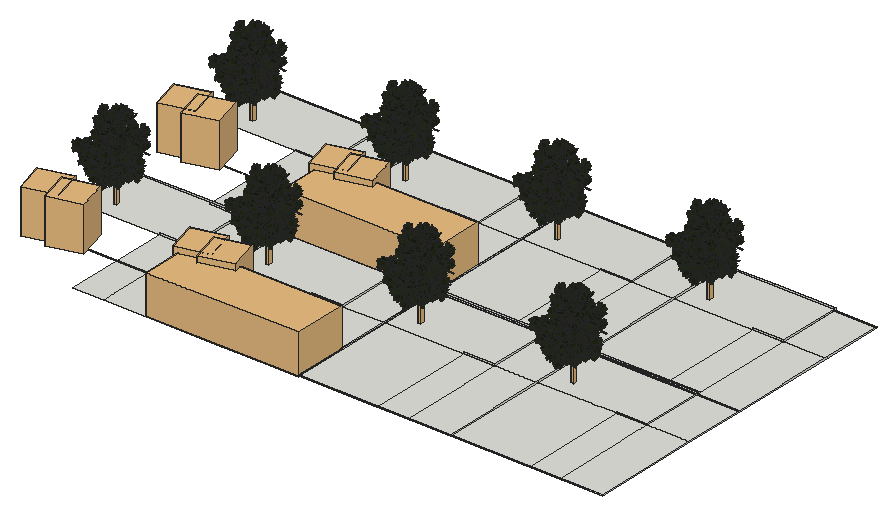
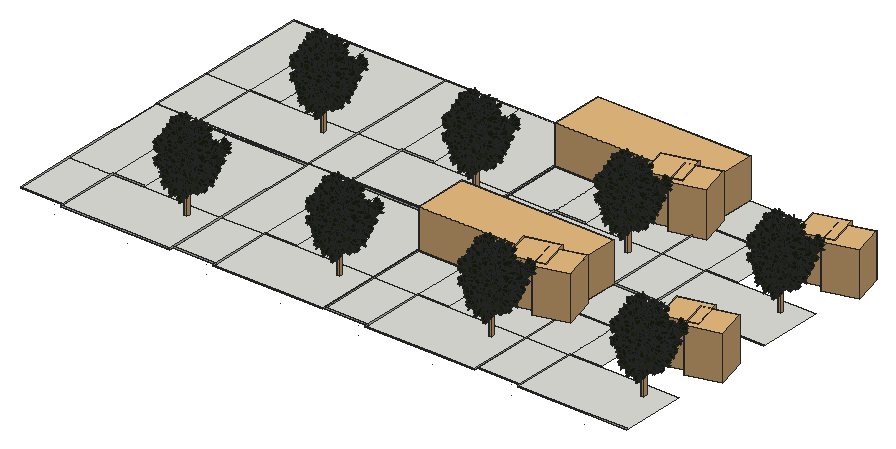
# SketchUp Ruby script. Lengths in inches.
U = 1.inch
M = Sketchup.active_model
def pt(a) = Geom::Point3d.new(a.map { |v| v * U })
def face(e, loops, mat)
  f = e.add_face(loops[0].map { |a| pt(a) })
  loops[1..].each { |l| e.add_face(l.map { |a| pt(a) }).erase! }
  f.material = f.back_material = mat if mat
  f
end
# faces: each face lists its corners as indices into pts; further lists are holes
def faces(e, pts, list, mat = nil) = list.each { |f| face(e, (f[0].is_a?(Array) ? f : [f]).map { |l| l.map { |i| pts[i] } }, mat) }
# xy, xz, yz: faces in a plane at the given z, y or x. An outline is a flat list of corners, or four numbers for a rectangle; further outlines are holes
def ring(l) = l.size == 4 ? [[l[0], l[1]], [l[2], l[1]], [l[2], l[3]], [l[0], l[3]]] : l.each_slice(2).to_a
def flat(e, list, mat, &to3) = list.each { |f| face(e, (f[0].is_a?(Array) ? f : [f]).map { |l| ring(l).map { |u, v| to3.(u, v) } }, mat) }
def xy(e, z, list, mat = nil) = flat(e, list, mat) { |x, y| [x, y, z] }
def xz(e, y, list, mat = nil) = flat(e, list, mat) { |x, z| [x, y, z] }
def yz(e, x, list, mat = nil) = flat(e, list, mat) { |y, z| [x, y, z] }
def lines(e, pts, list) = list.each { |a, b| e.add_line(pt(pts[a]), pt(pts[b])) }
# prism: a flat outline (further loops are holes) pulled along v
def prism(e, loops, v, mat = nil)
  f = face(e, loops, mat); d = Geom::Vector3d.new(v.map { |x| x * U })
  f.pushpull(f.normal.samedirection?(d) ? d.length : -d.length)
end
def box(e, o, s, mat = nil) = prism(e, [[o, [o[0] + s[0], o[1], o[2]], [o[0] + s[0], o[1] + s[1], o[2]], [o[0], o[1] + s[1], o[2]]]], [0, 0, s[2]], mat)
def at(x, y, z, deg = 0) = Geom::Transformation.translation(pt([x, y, z])) * Geom::Transformation.rotation(ORIGIN, Z_AXIS, deg.degrees)
def axes(o, x, y, z) = Geom::Transformation.new([*x, 0, *y, 0, *z, 0, *pt(o).to_a, 1])
def part(name) = M.definitions.add(name)
# library, detail: a bought-in or finely detailed component or shape, given as its bounding box
def library(name, o, s) = part(name).tap { |d| box(d.entities, o, s) }
def detail(e, o, s) = box(e.add_group.entities, o, s)
def put(e, d, t, mat = nil) = e.add_instance(d, t).tap { |i| i.material = mat if mat }
def group(e, t, mat = nil) = e.add_group.tap { |g| g.transformation = t; g.material = mat if mat }.entities
root = M.entities
M.materials.add("Green ash – green texture").color = [33, 41, 22]
M.materials.add("[Color_005]").color = [114, 114, 114]
M.materials.add("[Color_D09]").color = [86, 59, 49]
c1 = part("Component\#22")
xz(c1.entities,0,[[2.54,0,9.87,0.64,10.99,2.07,11.4,3.42,15.13,2.28,14.48,4.31,16.14,5.21,16.14,6.08,19.81,7.28,19.6,9.67,17.45,11.49,17.45,12.16,18.82,14.37,17.48,14.37,14.41,13.66,14.41,15.23,12.5625,17.49,9.84,15.21,8.9,13.85,7.74,13.625,7.35,12.68,6.87,13.02,6.35,12.27,5.92,10.47,4.2,7.42,2.84,6.89,0,2.38,0.07,1.59,2.8125,4.94,3.37,3.59,2.54,3.37,2.12,2.22]],"Green ash – green texture")
c2 = part("Component\#21")
xz(c2.entities,0,[[1.1,0,1.61,0,2.73,1.11,4.34,2.72,5.21,6.36,5.85,7.16,6.35,6.9375,6.85,8.05,8.03,8.05,8.625,9.25,10.11,11.7,9.56,13.83,9.56,15.84,7.83,15.84,6.03,14.37,5.31,16.54,4.4375,17.39,1.45,14.31,0,9.15,1.4,5.18,3.01,6.08,1.98,1.39]],"Green ash – green texture")
c3 = part("Component\#23")
put(c3.entities,c1,axes([0,7.77,0],[1,0,0],[0,0.89571,0.44464],[0,-0.44464,0.89571]))
put(c3.entities,c2,axes([2.15,6.37,5.26],[0.57629,-0.80824,0.12095],[0.79263,0.51673,-0.3236],[0.19905,0.28236,0.93843]))
c4 = part("Component\#24")
put(c4.entities,c3,axes([-4.97,-3.22,4.05],[0.69883,-0.69034,0.18725],[0.53248,0.3273,-0.7806],[0.47759,0.64522,0.59632]))
c5 = part("Component\#25")
put(c5.entities,c4,axes([0,5.2,2.2],[1,0,0],[0,0.90259,0.43051],[0,-0.43051,0.90259]))
c6 = part("leaf group 2")
put(c6.entities,c5,axes([-11.99,4.41,-4.35],[2.22014,-0.82385,1.14017],[1.36501,1.77637,-1.37441],[-0.33979,1.75315,1.92841]))
c7 = part("Component\#28")
put(c7.entities,c6,axes([-5.27,11.65,1.68],[-0.48323,0.10636,-0.43072],[-0.11515,-0.64511,-0.03012],[-0.42845,0.05342,0.49388]))
c8 = part("Component\#27")
xz(c8.entities,0,[[0.64,0,0,0.1875,4.21,2.81,8.59,4.11,12.8,4.11,19.57,2.81,12.8,3.73,8.59,3.73,4.21,2.3125]],"[Color_D09]")
c9 = part("Leafy twig \#1")
put(c9.entities,c7,axes([23.53,12.57,24.85],[0.06536,-0.90475,-0.42089],[0.61791,-0.2945,0.72901],[-0.78353,-0.30772,0.53981]))
put(c9.entities,c7,axes([22.7,12.25,24.83],[-0.47146,-0.89493,0.11311],[0.80135,-0.48549,-0.35888],[0.36776,-0.0521,0.90651]))
put(c9.entities,c7,axes([24.25,0.65,20.83],[0.8253,-0.50372,0.24924],[0.23848,0.71461,0.65749],[-0.51157,-0.48438,0.71194]))
put(c9.entities,c7,axes([23.54,-2.45,18.63],[0.04689,-0.92492,0.3511],[0.72122,-0.28285,-0.64421],[0.71641,0.2674,0.65188]))
put(c9.entities,c7,axes([22.39,16.15,27.04],[-0.5311,-0.82173,0.2419],[0.41574,0.01583,0.89559],[-0.77461,0.50499,0.40813]))
put(c9.entities,c8,axes([22.76,-5.09,13.48],[0,1.66539,0.44624],[-1.72414,0,0],[0,-0.44624,1.66539]))
c10 = part("Component\#26")
p = [[0,0,0.13],[0.41,0.77,0],[4.07,2.79,10.125],[3.73,2.15,10.23],[7.66,4.77,23.875],[7.4,4.27,23.96],
  [8.6875,5.26,35.99],[8.5,4.91,36.05],[8.32,4.9375,46.95],[8.21,4.74,46.98]]
faces(c10.entities,p,[[0,1,2,3],[3,2,4,5],[4,6,7,5],[6,8,9,7]],"[Color_005]")
c11 = part("Component\#30")
put(c11.entities,c10,axes([3.13,0.17,-0.45],[3.38032,6.88592,0.52481],[-5.85488,3.97559,0.303],[0,-1.35912,3.54524]))
put(c11.entities,c7,axes([0.37,31.375,148.94],[0.47772,0.64064,-1.51139],[2.85768,-0.62659,0.20284],[-0.43926,-3.3797,-0.3241]))
c12 = part("Leafy branch")
put(c12.entities,c9,axes([28.11,72.66,46.26],[0.77413,-0.41274,-0.47998],[0.6311,0.56229,0.53435],[0.04934,-0.71657,0.69577]))
put(c12.entities,c9,axes([31.25,3.94,9.17],[0.73236,0.67893,0.05208],[-0.46223,0.55185,-0.69413],[-0.5,0.48428,0.71797]))
put(c12.entities,c9,axes([20.16,84.84,57.95],[0.96628,0.19619,0.16678],[-0.2575,0.73909,0.62245],[-0.00115,-0.6444,0.76469]))
put(c12.entities,c9,axes([30.13,29.18,11.93],[0.86603,0.2796,0.41452],[0,0.82904,-0.55919],[-0.5,0.48428,0.71797]))
put(c12.entities,c9,axes([47.67,28.63,-3.7],[0.1205,-0.71255,0.69119],[0.96646,0.24327,0.08231],[-0.2268,0.65809,0.71797]))
put(c12.entities,c9,axes([48.76,50.64,76.31],[-0.6716,0.46861,-0.57389],[0.01402,0.78248,0.62252],[0.74078,0.41004,-0.53209]))
put(c12.entities,c11,axes([42.34,0,10.34],[0.39368,0,0],[0,0.22544,-0.24092],[0,0.54032,0.50562]))
put(c12.entities,c9,axes([64.51,80.82,101.08],[-0.99604,0.06562,-0.06004],[-0.0106,0.58266,0.81265],[0.08831,0.81006,-0.57966]))
c13 = library("Component\#31",[-6.35,9.4375,-76.57],[12.56,13.68,315.77])
c14 = part("Component\#33")
put(c14.entities,c9,axes([-3.64,36.17,23.18],[0.95801,0.10249,0.26779],[-0.28581,0.41631,0.86313],[-0.02302,-0.90343,0.42812]))
put(c14.entities,c9,axes([13.16,55.79,39.92],[0.70711,-0.61725,0.34497],[0,0.48786,0.87292],[-0.70711,-0.61725,0.34497]))
put(c14.entities,c11,axes([18.8125,5.17,0.46],[0.25503,0,0],[0,0.20007,-0.0752],[0,0.16866,0.44872]))
put(c14.entities,c9,axes([23.62,-10.17,21.5],[-0.56253,0.81775,0.12181],[0.38738,0.13053,0.91263],[0.73041,0.56057,-0.39021]))
put(c14.entities,c9,axes([45.18,27.18,68.96],[-0.96593,-0.22593,0.12627],[0.12295,0.02876,0.992],[-0.22775,0.97372,0]))
c15 = part("Component\#32")
put(c15.entities,c11,axes([21.47,3.93,0.22],[0.25503,0,0],[0,0.21068,-0.03601],[0,0.08077,0.47252]))
put(c15.entities,c9,axes([-4.05,13.6875,55.34],[0.70711,0.70373,-0.069],[0,0.09758,0.99523],[0.70711,-0.70373,0.069]))
put(c15.entities,c9,axes([6.52,33.54,18.07],[0.92587,-0.37604,0.03687],[0,0.09758,0.99523],[-0.37784,-0.92145,0.09035]))
c16 = part("Leafy branch \#1")
put(c16.entities,c9,axes([26.17,74.02,40.56],[0.25882,-0.64004,0.72344],[0,0.74896,0.66262],[-0.96593,-0.1715,0.19384]))
put(c16.entities,c9,axes([6.38,24.03,55.81],[-0.04786,0.8645,-0.50035],[0.15558,0.50126,0.85119],[0.98666,-0.03711,-0.15849]))
put(c16.entities,c11,axes([17.68,0,1.01],[0.32282,0,0],[0,0.21407,-0.16545],[0,0.37107,0.48011]))
put(c16.entities,c9,axes([-9.1875,31.15,28.07],[0.82314,0.37626,-0.42529],[0,0.74896,0.66262],[0.56784,-0.54543,0.61649]))
put(c16.entities,c9,axes([0.54,-12.07,9.94],[0.19622,0.90478,-0.37799],[-0.67396,0.40444,0.61823],[0.71224,0.13344,0.68914]))
put(c16.entities,c9,axes([7.34,9.15,39.57],[0.05153,0.73872,-0.67204],[0.38679,0.60565,0.6954],[0.92072,-0.29578,-0.25452]))
put(c16.entities,c9,axes([36.2,51.23,15.73],[-0.18626,-0.35374,0.91661],[-0.31641,0.90483,0.2849],[-0.93016,-0.23696,-0.28046]))
c17 = part("Tree")
put(c17.entities,c12,axes([-22.29,52.36,216.76],[0.38964,-1.07313,-0.10036],[1.06809,0.37236,0.19631],[-0.13881,-0.14712,1.22884]))
put(c17.entities,c12,axes([59.83,6.78,230.57],[-1.28826,-0.23008,-0.3647],[0.05148,-1.22938,0.51215],[-0.34663,0.55136,1.25774]))
put(c17.entities,c13,axes([-2.16,-18.04,104.22],[1.30157,0,0],[0,1.30157,0],[0,0,1.36111]))
put(c17.entities,c12,axes([-55.8,4.2,115.32],[1.30157,0,0],[0,1.29536,0.19359],[0,-0.26855,1.38538]))
put(c17.entities,c12,axes([5.36,-52.22,156.04],[-0.23532,1.19719,-0.71362],[-1.32974,0,0.39335],[0.40758,0.6912,1.23603]))
put(c17.entities,c14,axes([-20.09,22.57,317.7],[0,-1.33697,0],[1.33697,0,0],[0,0,1.4573]))
put(c17.entities,c12,axes([44.2,-31.84,172.82],[-1.11894,0.85085,0],[-0.85085,-1.11894,0],[0,0,1.53221]))
put(c17.entities,c12,axes([-10.2,63.7,119.93],[0.28716,-1.46366,0],[1.41378,0.27737,0.38604],[-0.41292,-0.08101,1.5704]))
put(c17.entities,c12,axes([-29.03,-40.72,232.79],[0.5211,0.98898,-0.38718],[-1.02974,0.58664,0.11255],[0.35577,0.28216,1.19957]))
put(c17.entities,c12,axes([44.92,21.7,135.38],[-1.05627,-0.44294,0],[0.44294,-1.05627,0],[0,0,1.24847]))
put(c17.entities,c14,axes([-32.94,-0.59,304.82],[1.2814,-0.22825,0],[0.22825,1.2814,0],[0,0,1.41871]))
put(c17.entities,c14,axes([0.6,-31.29,315.98],[0.13082,1.33422,0],[-1.33422,0.13082,0],[0,0,1.46127]))
put(c17.entities,c14,axes([21.3,1.66,315.16],[-1.25722,0.32198,-0.09905],[-0.32539,-1.26867,0.00612],[-0.08719,0.09194,1.40547]))
put(c17.entities,c15,axes([-19,30.84,372.72],[0.65078,-1.12719,0],[1.12719,0.65078,0],[0,0,1.41871]))
put(c17.entities,c15,axes([14.39,-16.125,357],[-0.73695,1.06095,0.15933],[-1.03698,-0.75397,0.2242],[0.29981,0,1.38667]))
put(c17.entities,c16,axes([-5.9,-20.03,270.39],[0,1.47598,0],[-1.4157,0,0.41751],[0.45509,0,1.54311]))
put(c17.entities,c16,axes([-18.4375,22.18,263.88],[0.84243,-1.42226,-0.32685],[1.40385,0.7063,0.64743],[-0.37678,-0.54841,1.68147]))
put(c17.entities,c16,axes([-29.32,4.9,283.41],[1.35363,0,0],[0,1.33841,0.20242],[0,-0.22063,1.45887]))
put(c17.entities,c16,axes([17.31,11.65,257.52],[-1.14969,-0.5642,-0.25322],[0.46017,-1.12719,0.50159],[-0.40066,0.32434,1.3027]))
put(c17.entities,c16,axes([16.3,15.3125,240.45],[-0.98541,-0.85203,0.68095],[1.00747,-1.01506,0.22317],[0.31818,0.5753,1.40228]))
put(c17.entities,c12,axes([-46.75,22.93,206.12],[1.08363,-0.37101,0],[0.37101,1.08363,0],[0,0,1.24847]))
put(c17.entities,c12,axes([41.1,-35.18,99.125],[-1.05556,0.85173,0.25344],[-0.84493,-1.04965,0.12953],[0.39153,-0.09409,1.38106]))
c18 = library("BPJ-Road5D",[0,0,1],[442,720,229.125])
c19 = library("Palm tree",[-4.09,-4.52,0],[193.52,193.51,258.93])
c20 = part("Palm+Tree")
put(c20.entities,c19,at(25.51,-21.81,0,15))
xy(root,-26.92,[[491.71,2.31,671.36,638.99],[671.36,2.31,923.05,638.99],[923.05,2.31,1384.3,638.99],[1384.3,2.31,1563.95,638.99],[1563.95,2.31,1815.63,638.99],
  [30.46,638.99,30.46,1021.31,491.71,1021.31,491.71,1001.66,671.36,1001.66,671.36,638.99],[671.36,638.99,923.05,1001.66],[923.05,638.99,1563.95,1001.66],[1563.95,638.99,1815.63,1001.66],[491.71,1001.66,671.36,1021.31],
  [671.36,1001.66,923.05,1638.35],[923.05,1001.66,1384.3,1021.31],[1384.3,1001.66,1563.95,1021.31],[1563.95,1001.66,1815.63,1638.35],[491.71,1021.31,671.36,1638.35],
  [923.05,1021.31,1384.3,1638.35],[1384.3,1021.31,1563.95,1638.35],[30.46,1638.35,671.36,2020.66],[671.36,1638.35,923.05,2001.02],[923.05,1638.35,1563.95,2020.66],
  [1563.95,1638.35,1815.63,2001.02]])
xy(root,-23.23,[[923.05,2.31,1815.63,317.81],[923.05,1001.66,1815.63,1317.16]])
xy(root,-22.23,[[1815.63,0,2276.89,636.6875],[2276.89,0,2456.54,636.6875],[2456.54,0,2708.22,636.6875],[2708.22,0,3169.48,636.6875],[3169.48,0,3349.13,636.6875],
  [3349.13,0,3600.8125,636.6875],[1815.63,636.6875,2456.54,999.35],[2456.54,636.6875,2708.22,999.35],[2708.22,636.6875,3349.13,999.35],[3349.13,636.6875,3600.8125,999.35],
  [1815.63,999.35,2276.89,1019],[2276.89,999.35,2456.54,1019],[2456.54,999.35,2708.22,1636.04],[2708.22,999.35,3169.48,1019],[3169.48,999.35,3349.13,1019],
  [3349.13,999.35,3600.8125,1636.04],[1815.63,1019,2276.89,1636.04],[2276.89,1019,2456.54,1636.04],[2708.22,1019,3169.48,1636.04],[3169.48,1019,3349.13,1636.04],
  [1815.63,1636.04,2456.54,2018.36],[2456.54,1636.04,2708.22,1998.71],[2708.22,1636.04,3349.13,2018.36],[3349.13,1636.04,3600.8125,1998.71]])
xz(root,0,[[1815.63,-22.23,2708.22,-18.54],[2708.22,-22.23,3600.8125,-18.54]])
xz(root,2.31,[[923.05,-26.92,1815.63,-23.23]])
xz(root,317.81,[[30.46,-23.23,923.05,-19.54],[923.05,-23.23,1815.63,-19.54]])
xz(root,636.6875,[[2276.89,-22.23,2456.54,-14.85],[3169.48,-22.23,3349.13,-14.85]])
xz(root,638.99,[[491.71,-26.92,671.36,-19.54],[1384.3,-26.92,1563.95,-19.54]])
xz(root,999.35,[[1815.63,-22.23,2456.54,-18.54],[2456.54,-22.23,2708.22,-18.54],[2708.22,-22.23,3349.13,-18.54],[3349.13,-22.23,3600.8125,-18.54]])
xz(root,1001.66,[[671.36,-26.92,923.05,-19.54],[923.05,-26.92,1563.95,-23.23],[1563.95,-26.92,1815.63,-23.23],[1563.95,-23.23,1815.63,-19.54]])
xz(root,1019,[[1815.63,-22.23,2097.23,-14.85],[2097.23,-22.23,2456.54,-14.85],[2708.22,-22.23,2989.82,-14.85],[2989.82,-22.23,3349.13,-14.85]])
xz(root,1021.31,[[30.46,-26.92,312.05,-19.54],[312.05,-26.92,671.36,-19.54],[923.05,-26.92,1204.64,-19.54],[1204.64,-26.92,1563.95,-19.54]])
xz(root,1317.16,[[30.46,-23.23,923.05,-19.54],[923.05,-23.23,1815.63,-19.54]])
xz(root,1636.04,[[2276.89,-22.23,2456.54,-14.85],[3169.48,-22.23,3349.13,-14.85]])
xz(root,1638.35,[[491.71,-26.92,671.36,-19.54],[1384.3,-26.92,1563.95,-19.54]])
xz(root,1998.71,[[2456.54,-22.23,2708.22,-14.85],[3349.13,-22.23,3600.8125,-14.85]])
xz(root,2001.02,[[671.36,-26.92,923.05,-19.54],[1563.95,-26.92,1815.63,-19.54]])
xz(root,2018.36,[[1815.63,-22.23,2097.23,-14.85],[2097.23,-22.23,2456.54,-14.85],[2708.22,-22.23,2989.82,-14.85],[2989.82,-22.23,3349.13,-14.85]])
xz(root,2020.66,[[30.46,-26.92,312.05,-19.54],[312.05,-26.92,671.36,-19.54],[923.05,-26.92,1204.64,-19.54],[1204.64,-26.92,1563.95,-19.54]])
yz(root,671.36,[[638.99,-26.92,1001.66,-19.54],[1001.66,-26.92,1021.31,-19.54],[1638.35,-26.92,2001.02,-19.54],[2001.02,-26.92,2020.66,-19.54]])
yz(root,923.05,[[2.31,-26.92,2.31,-23.23,317.81,-23.23,317.81,-19.54,638.99,-19.54,638.99,-26.92],[638.99,-26.92,1001.66,-19.54],[1001.66,-26.92,1021.31,-23.23],[1021.31,-26.92,1021.31,-23.23,1317.16,-23.23,1317.16,-19.54,1638.35,-19.54,1638.35,-26.92],[1638.35,-26.92,2001.02,-19.54],
  [2001.02,-26.92,2020.66,-19.54],[1001.66,-23.23,1021.31,-19.54]])
yz(root,1563.95,[[638.99,-26.92,1001.66,-19.54],[1001.66,-26.92,1021.31,-19.54],[1638.35,-26.92,2001.02,-19.54],[2001.02,-26.92,2020.66,-19.54]])
yz(root,1815.63,[[2.31,-26.92,638.99,-26.92,638.99,-22.23,317.81,-22.23,317.81,-23.23,2.31,-23.23],[638.99,-26.92,1001.66,-22.23],[1001.66,-26.92,1638.35,-26.92,1638.35,-22.23,1317.16,-22.23,1317.16,-23.23,1001.66,-23.23],[1638.35,-26.92,2001.02,-22.23],[0,-22.23,0,-18.54,315.5,-18.54,315.5,-14.85,1019,-14.85,1019,-18.54,999.35,-18.54,999.35,-19.54,317.81,-19.54,317.81,-22.23],
  [317.81,-22.23,638.99,-19.54],[638.99,-22.23,999.35,-19.54],[1001.66,-22.23,1001.66,-19.54,999.35,-19.54,999.35,-18.54,1019,-18.54,1019,-22.23],[999.35,-22.23,1001.66,-19.54],[1019,-22.23,1019,-18.54,1314.85,-18.54,1314.85,-14.85,2018.36,-14.85,2018.36,-22.23,2001.02,-22.23,2001.02,-19.54,1317.16,-19.54,1317.16,-22.23],
  [1317.16,-22.23,1638.35,-19.54],[1638.35,-22.23,2001.02,-19.54]])
yz(root,2456.54,[[636.6875,-22.23,999.35,-14.85],[999.35,-22.23,1019,-14.85],[1636.04,-22.23,1998.71,-14.85],[1998.71,-22.23,2018.36,-14.85]])
yz(root,2708.22,[[0,-22.23,0,-18.54,315.5,-18.54,315.5,-14.85,636.6875,-14.85,636.6875,-22.23],[636.6875,-22.23,999.35,-14.85],[999.35,-22.23,1019,-18.54],[1019,-22.23,1019,-18.54,1314.85,-18.54,1314.85,-14.85,1636.04,-14.85,1636.04,-22.23],[1636.04,-22.23,1998.71,-14.85],
  [1998.71,-22.23,2018.36,-14.85]])
yz(root,3349.13,[[636.6875,-22.23,999.35,-14.85],[999.35,-22.23,1019,-14.85],[1636.04,-22.23,1998.71,-14.85],[1998.71,-22.23,2018.36,-14.85]])
yz(root,3600.8125,[[0,-22.23,636.6875,-22.23,636.6875,-14.85,315.5,-14.85,315.5,-18.54,0,-18.54],[636.6875,-22.23,999.35,-14.85],[999.35,-22.23,1636.04,-22.23,1636.04,-14.85,1314.85,-14.85,1314.85,-18.54,999.35,-18.54],[1636.04,-22.23,1998.71,-14.85]])
p = [[2494.04,1019,-24.0625],[2494.04,1019.06,-24.0625],[2494.04,1019,-79.41],[2494.04,1019.06,-79.41],[2064.92,1019,-79.41],[2064.92,1019.06,-79.41],
  [3386.63,1019,-24.0625],[3386.63,1019.06,-24.0625],[3386.63,1019,-79.41],[3386.63,1019.06,-79.41],[2957.51,1019,-79.41],[2957.51,1019.06,-79.41],
  [708.86,1021.31,-28.75],[708.86,1021.37,-28.75],[708.86,1021.31,-84.1],[708.86,1021.37,-84.1],[279.74,1021.31,-84.1],[279.74,1021.37,-84.1],
  [1601.45,1021.31,-28.75],[1601.45,1021.37,-28.75],[1601.45,1021.31,-84.1],[1601.45,1021.37,-84.1],[1172.33,1021.31,-84.1],[1172.33,1021.37,-84.1],
  [2494.04,2018.36,-24.0625],[2494.04,2018.42,-24.0625],[2494.04,2018.36,-79.41],[2494.04,2018.42,-79.41],[2064.92,2018.36,-79.41],[2064.92,2018.42,-79.41],
  [3386.63,2018.36,-24.0625],[3386.63,2018.42,-24.0625],[3386.63,2018.36,-79.41],[3386.63,2018.42,-79.41],[2957.51,2018.36,-79.41],[2957.51,2018.42,-79.41],
  [708.86,2020.66,-84.1],[708.86,2020.73,-84.1],[279.74,2020.66,-84.1],[279.74,2020.73,-84.1],[708.86,2020.66,-28.75],[708.86,2020.73,-28.75],
  [1601.45,2020.66,-28.75],[1601.45,2020.73,-28.75],[1172.33,2020.66,-84.1],[1172.33,2020.73,-84.1],[1601.45,2020.66,-84.1],[1601.45,2020.73,-84.1]]
lines(root,p,[[0,1],[2,3],[4,5],[6,7],[8,9],[10,11],[12,13],[14,15],[16,17],[18,19],[20,21],[22,23],
  [24,25],[26,27],[28,29],[30,31],[32,33],[34,35],[36,37],[38,39],[40,41],[42,43],[44,45],[46,47]])
put(root,c17,at(165.7,729.1,-19.54))
put(root,c17,at(165.7,1728.45,-19.54))
put(root,c17,at(1058.29,729.1,-19.54))
put(root,c17,at(1058.29,1728.45,-19.54))
put(root,c17,at(1950.88,1726.15,-14.85))
put(root,c17,at(1950.88,726.79,-14.85))
put(root,c17,at(2843.47,726.79,-14.85))
put(root,c17,at(2843.47,1726.15,-14.85))
put(root,c18,axes([1815.63,999.35,-23.23],[0,0.71,0],[-1.23971,0,0],[0,0,1]))
put(root,c18,axes([1815.63,0,-23.23],[0,0.71,0],[-1.23971,0,0],[0,0,1]))
put(root,c20,at(-16.75,1252.45,-22.2))
put(root,c20,at(-16.75,253.09,-22.2))
put(root,c20,at(875.84,1252.45,-22.2))
put(root,c20,at(875.84,253.09,-22.2))
put(root,c20,at(127.84,1250.42,-20.89))
put(root,c20,at(127.84,251.0625,-20.89))
put(root,c20,at(1020.43,1250.42,-20.89))
put(root,c20,at(1020.43,251.0625,-20.89))
